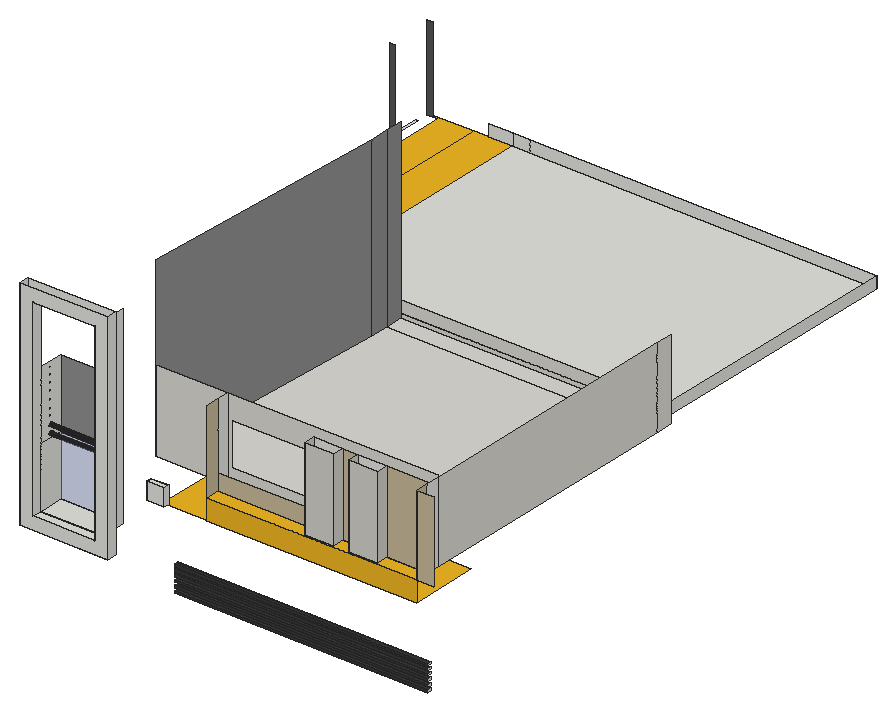
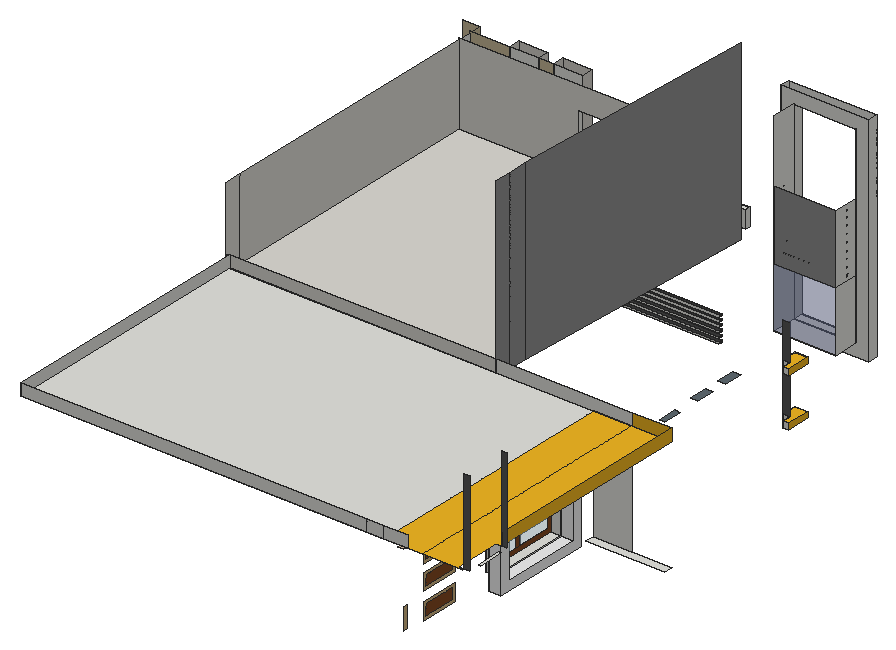
# SketchUp Ruby script. Lengths in inches.
U = 1.inch
M = Sketchup.active_model
def pt(a) = Geom::Point3d.new(a.map { |v| v * U })
def face(e, loops, mat)
  f = e.add_face(loops[0].map { |a| pt(a) })
  loops[1..].each { |l| e.add_face(l.map { |a| pt(a) }).erase! }
  f.material = f.back_material = mat if mat
  f
end
# faces: each face lists its corners as indices into pts; further lists are holes
def faces(e, pts, list, mat = nil) = list.each { |f| face(e, (f[0].is_a?(Array) ? f : [f]).map { |l| l.map { |i| pts[i] } }, mat) }
# xy, xz, yz: faces in a plane at the given z, y or x. An outline is a flat list of corners, or four numbers for a rectangle; further outlines are holes
def ring(l) = l.size == 4 ? [[l[0], l[1]], [l[2], l[1]], [l[2], l[3]], [l[0], l[3]]] : l.each_slice(2).to_a
def flat(e, list, mat, &to3) = list.each { |f| face(e, (f[0].is_a?(Array) ? f : [f]).map { |l| ring(l).map { |u, v| to3.(u, v) } }, mat) }
def xy(e, z, list, mat = nil) = flat(e, list, mat) { |x, y| [x, y, z] }
def xz(e, y, list, mat = nil) = flat(e, list, mat) { |x, z| [x, y, z] }
def yz(e, x, list, mat = nil) = flat(e, list, mat) { |y, z| [x, y, z] }
def lines(e, pts, list) = list.each { |a, b| e.add_line(pt(pts[a]), pt(pts[b])) }
# prism: a flat outline (further loops are holes) pulled along v
def prism(e, loops, v, mat = nil)
  f = face(e, loops, mat); d = Geom::Vector3d.new(v.map { |x| x * U })
  f.pushpull(f.normal.samedirection?(d) ? d.length : -d.length)
end
def box(e, o, s, mat = nil) = prism(e, [[o, [o[0] + s[0], o[1], o[2]], [o[0] + s[0], o[1] + s[1], o[2]], [o[0], o[1] + s[1], o[2]]]], [0, 0, s[2]], mat)
def at(x, y, z, deg = 0) = Geom::Transformation.translation(pt([x, y, z])) * Geom::Transformation.rotation(ORIGIN, Z_AXIS, deg.degrees)
def axes(o, x, y, z) = Geom::Transformation.new([*x, 0, *y, 0, *z, 0, *pt(o).to_a, 1])
def part(name) = M.definitions.add(name)
# library, detail: a bought-in or finely detailed component or shape, given as its bounding box
def library(name, o, s) = part(name).tap { |d| box(d.entities, o, s) }
def detail(e, o, s) = box(e.add_group.entities, o, s)
def put(e, d, t, mat = nil) = e.add_instance(d, t).tap { |i| i.material = mat if mat }
def group(e, t, mat = nil) = e.add_group.tap { |g| g.transformation = t; g.material = mat if mat }.entities
root = M.entities
M.materials.add("[0045_Goldenrod]").color = [239, 181, 35]
M.materials.add("[Carrera Marble]").color = [239, 239, 239]
M.materials.add("[Color M04]").color = [142, 142, 142]
M.materials.add("[Color M06]").color = [86, 86, 86]
M.materials.add("[Color M07]").color = [58, 58, 58]
M.materials.add("[Formica Laminate Light]").color = [213, 189, 164]
M.materials.add("[Formica Speckled Grey]").color = [94, 105, 111]
M.materials.add("[Quartz Light Brown]").color = [199, 184, 152]
M.materials.add("[Terrazzo Tile Light]").color = [219, 217, 210]
M.materials.add("[Tile Travertine 2 inch]").color = [211, 208, 201]
M.materials.add("[Translucent Glass Safety]").color = [204, 235, 244]
M.materials["[Translucent Glass Safety]"].alpha = 0.5
M.materials.add("[Translucent Glass Sky Reflection]").color = [126, 138, 183]
M.materials["[Translucent Glass Sky Reflection]"].alpha = 0.52
M.materials.add("[Wood Cherry Original]").color = [130, 73, 35]
M.materials.add("[Wood Floor Light]").color = [204, 176, 127]
box(root,[220.22,108.25,362.15],[19.63,5.9375,19.63])
xy(root,255.625,[[8.375,483.625,97.02,493.85]])
xy(root,256.33,[[226.34,139.81,513.45,143.95]])
xy(root,258.89,[[226.34,139.81,513.45,143.95]],"[Color M07]")
xy(root,261.64,[[226.34,139.81,513.45,143.95]])
xy(root,264.2,[[226.34,139.81,513.45,143.95]],"[Color M07]")
xy(root,265.95,[[82.9,518.89,97.02,632.14]],"[Carrera Marble]")
xy(root,267.45,[[226.34,139.81,513.45,143.95]])
xy(root,270.02,[[226.34,139.81,513.45,143.95]],"[Color M07]")
xy(root,273.08,[[226.34,139.81,513.45,143.95]])
xy(root,275.64,[[226.34,139.81,513.45,143.95]],"[Color M07]")
xy(root,276.41,[[97.02,529.35,108.15,621.68]])
xy(root,276.41,[[82.9,529.35,97.02,621.68]],"[Carrera Marble]")
xy(root,278.27,[[226.34,139.81,513.45,143.95]])
xy(root,280.83,[[226.34,139.81,513.45,143.95]],"[Color M07]")
xy(root,283.14,[[226.34,139.81,513.45,143.95]])
xy(root,283.375,[[73.3,112.625,172.24,123.625]])
xy(root,285.7,[[226.34,139.81,513.45,143.95]],"[Color M07]")
xy(root,295.16,[[38.625,253.03,38.625,280.03,45.3125,280.03,45.3125,270.46,53.375,270.46,53.375,253.03]],"[0045_Goldenrod]")
xy(root,297.39,[[87.31,112.625,158.23,123.625],[87.31,123.625,158.23,152]])
xy(root,301.97,[[38.625,253.03,53.375,253.03,53.375,270.46,45.3125,270.46,45.3125,280.03,38.625,280.03]],"[0045_Goldenrod]")
xy(root,350.16,[[38.625,253.03,38.625,280.03,45.3125,280.03,45.3125,270.46,53.375,270.46,53.375,253.03]],"[0045_Goldenrod]")
xy(root,354.51,[[226.34,123.625,513.45,200.74]],"[0045_Goldenrod]")
xy(root,356.97,[[38.625,253.03,53.375,253.03,53.375,270.46,45.3125,270.46,45.3125,280.03,38.625,280.03]],"[0045_Goldenrod]")
xy(root,358.98,[[82.9,529.35,97.02,621.68],[97.02,529.35,108.15,621.68]])
xy(root,360.75,[[97.02,660.4,103.59,752.02]],"[Formica Laminate Light]")
xy(root,367.23,[[53.375,329.31,62.1875,350.56],[53.375,368.62,61.9375,389.87],[53.375,415.62,59.375,436.87]],"[Formica Speckled Grey]")
xy(root,369.45,[[82.9,518.89,97.02,632.14]],"[Carrera Marble]")
xy(root,378,[[435.42,123.625,467.86,125.375],[385.17,125.375,418.48,138.52],[435.42,125.375,467.86,138.52],[276.16,138.52,513.45,153.42]])
xy(root,378,[[276.16,123.625,435.42,123.625,435.42,138.52,418.48,138.52,418.48,125.375,385.17,125.375,385.17,138.52,276.16,138.52],[467.86,123.625,513.45,138.52]],"[0045_Goldenrod]")
xy(root,378,[[194.63,153.42,513.45,153.42,513.45,463.7,208.03,463.7,208.03,442.17],[208.03,463.7,513.45,483.625]],"[Terrazzo Tile Light]")
xy(root,383.375,[[97.02,483.625,509.21,779.875]])
xy(root,383.375,[[8.375,483.625,8.375,724.47,14.37,724.47,14.37,777.2,8.375,777.2,8.375,779.875,53.375,779.875,53.375,483.625],[53.375,483.625,97.02,779.875]],"[0045_Goldenrod]")
xy(root,383.48,[[0,735.45,2.5625,763.82]])
xz(root,112.625,[[[73.3,283.375,172.24,529.3125],[87.31,297.39,158.23,515.31]]])
xz(root,123.625,[[[73.3,283.375,172.24,529.3125],[87.31,297.39,158.23,515.31]]])
xz(root,123.625,[[276.16,354.51,513.45,378]],"[0045_Goldenrod]")
xz(root,123.625,[[513.45,378,533.375,468.5]],"[Quartz Light Brown]")
xz(root,125.375,[[385.17,378,418.48,471],[435.42,378,467.86,471]],"[Tile Travertine 2 inch]")
xz(root,138.52,[[385.17,378,418.48,471],[435.42,378,467.86,471]])
xz(root,138.52,[[276.16,378,385.17,396.69],[418.48,378,435.42,471],[467.86,378,513.45,471]],"[Quartz Light Brown]")
xz(root,139.81,[[226.34,256.33,513.45,258.89],[226.34,261.64,513.45,264.2],[226.34,267.45,513.45,270.02],[226.34,273.08,513.45,275.64],[226.34,278.27,513.45,280.83],
  [226.34,283.14,513.45,285.7]],"[Color M07]")
xz(root,143.95,[[226.34,256.33,513.45,258.89],[226.34,261.64,513.45,264.2],[226.34,267.45,513.45,270.02],[226.34,273.08,513.45,275.64],[226.34,278.27,513.45,280.83],
  [226.34,283.14,513.45,285.7]])
xz(root,152,[[87.31,365.69,158.23,444.16]],"[Color M04]")
xz(root,152,[[87.31,297.39,158.23,365.69]],"[Translucent Glass Sky Reflection]")
xz(root,153.42,[[194.63,378,276.16,471],[[276.16,378,513.45,471],[280.22,396.69,379.09,445.19]]],"[Terrazzo Tile Light]")
xz(root,253.03,[[38.625,295.16,53.375,301.97],[38.625,350.16,53.375,356.97]],"[0045_Goldenrod]")
xz(root,270.46,[[45.3125,295.16,53.375,301.97],[45.3125,350.16,53.375,356.97]])
xz(root,270.46,[[45.3125,301.97,53.375,350.16],[45.3125,356.97,53.375,397.66]],"[Color M06]")
xz(root,280.03,[[38.625,295.16,45.3125,301.97],[38.625,350.16,45.3125,356.97]])
xz(root,483.625,[[53.375,255.625,97.02,383.375],[509.21,378,513.45,396.875],[53.375,383.375,208.03,396.875]])
xz(root,483.625,[[8.375,383.375,53.375,396.875]],"[0045_Goldenrod]")
xz(root,483.625,[[208.03,378,509.21,383.375],[208.03,383.375,509.21,396.875]],"[Terrazzo Tile Light]")
xz(root,518.89,[[82.9,265.95,97.02,369.45]],"[Carrera Marble]")
xz(root,529.35,[[97.02,276.41,108.15,358.98]])
xz(root,529.35,[[82.9,276.41,97.02,358.98]],"[Carrera Marble]")
xz(root,621.68,[[97.02,276.41,108.15,358.98]])
xz(root,621.68,[[82.9,276.41,97.02,358.98]],"[Carrera Marble]")
xz(root,632.14,[[82.9,265.95,97.02,369.45]],"[Carrera Marble]")
xz(root,724.47,[[2.5625,383.375,8.375,479.1875]],"[Color M06]")
xz(root,777.2,[[2.5625,383.375,8.375,479.1875]],"[Color M06]")
xz(root,779.875,[[70.21,383.375,97.02,396.875],[97.02,383.375,116.75,396.875],[116.75,383.375,509.21,396.875]])
yz(root,8.375,[[483.625,383.375,724.47,396.875]],"[0045_Goldenrod]")
yz(root,38.625,[[253.03,295.16,280.03,301.97],[253.03,350.16,280.03,356.97]],"[0045_Goldenrod]")
yz(root,45.3125,[[270.46,295.16,280.03,301.97],[270.46,350.16,280.03,356.97]])
yz(root,53.375,[[253.03,295.16,270.46,301.97],[253.03,350.16,270.46,356.97]])
yz(root,73.3,[[112.625,283.375,123.625,529.3125]])
yz(root,82.9,[[[518.89,265.95,632.14,369.45],[529.35,276.41,621.68,358.98]]],"[Carrera Marble]")
yz(root,87.31,[[112.625,297.39,123.625,515.31],[123.625,297.39,152,365.69],[[123.625,365.69,152,444.16],[136.99,436.55,136.55,436.61,136.14,436.78,135.79,437.05,135.52,437.4,135.36,437.81,135.3,438.24,135.36,438.68,135.52,439.09,135.79,439.44,136.14,439.7,136.55,439.87,136.99,439.93,137.42,439.87,137.83,439.7,138.18,439.44,138.45,439.09,138.62,438.68,138.67,438.24,138.62,437.81,138.45,437.4,138.18,437.05,137.83,436.78,137.42,436.61],[136.99,369.93,136.55,369.99,136.14,370.16,135.79,370.42,135.52,370.77,135.36,371.18,135.3,371.62,135.36,372.05,135.52,372.46,135.79,372.81,136.14,373.08,136.55,373.25,136.99,373.3,137.42,373.25,137.83,373.08,138.18,372.81,138.45,372.46,138.62,372.05,138.67,371.62,138.62,371.18,138.45,370.77,138.18,370.42,137.83,370.16,137.42,369.99],[136.99,429.05,136.55,429.11,136.14,429.28,135.79,429.55,135.52,429.9,135.36,430.31,135.3,430.74,135.36,431.18,135.52,431.59,135.79,431.94,136.14,432.2,136.55,432.37,136.99,432.43,137.42,432.37,137.83,432.2,138.18,431.94,138.45,431.59,138.62,431.18,138.67,430.74,138.62,430.31,138.45,429.9,138.18,429.55,137.83,429.28,137.42,429.11],[136.99,378.62,136.55,378.67,136.14,378.84,135.79,379.11,135.52,379.46,135.36,379.87,135.3,380.3,135.36,380.74,135.52,381.15,135.79,381.5,136.14,381.77,136.55,381.93,136.99,381.99,137.42,381.93,137.83,381.77,138.18,381.5,138.45,381.15,138.62,380.74,138.67,380.3,138.62,379.87,138.45,379.46,138.18,379.11,137.83,378.84,137.42,378.67],[136.99,420.74,136.55,420.8,136.14,420.97,135.79,421.24,135.52,421.59,135.36,421.99,135.3,422.43,135.36,422.87,135.52,423.27,135.79,423.62,136.14,423.89,136.55,424.06,136.99,424.12,137.42,424.06,137.83,423.89,138.18,423.62,138.45,423.27,138.62,422.87,138.67,422.43,138.62,421.99,138.45,421.59,138.18,421.24,137.83,420.97,137.42,420.8],[136.99,387.18,136.55,387.24,136.14,387.41,135.79,387.67,135.52,388.02,135.36,388.43,135.3,388.87,135.36,389.3,135.52,389.71,135.79,390.06,136.14,390.33,136.55,390.5,136.99,390.55,137.42,390.5,137.83,390.33,138.18,390.06,138.45,389.71,138.62,389.3,138.67,388.87,138.62,388.43,138.45,388.02,138.18,387.67,137.83,387.41,137.42,387.24],[136.99,412.55,136.55,412.61,136.14,412.78,135.79,413.05,135.52,413.4,135.36,413.81,135.3,414.24,135.36,414.68,135.52,415.09,135.79,415.44,136.14,415.7,136.55,415.87,136.99,415.93,137.42,415.87,137.83,415.7,138.18,415.44,138.45,415.09,138.62,414.68,138.67,414.24,138.62,413.81,138.45,413.4,138.18,413.05,137.83,412.78,137.42,412.61],[136.99,394.8,136.55,394.86,136.14,395.03,135.79,395.3,135.52,395.65,135.36,396.06,135.3,396.49,135.36,396.93,135.52,397.34,135.79,397.69,136.14,397.95,136.55,398.12,136.99,398.18,137.42,398.12,137.83,397.95,138.18,397.69,138.45,397.34,138.62,396.93,138.67,396.49,138.62,396.06,138.45,395.65,138.18,395.3,137.83,395.03,137.42,394.86],[136.99,403.55,136.55,403.61,136.14,403.78,135.79,404.05,135.52,404.4,135.36,404.81,135.3,405.24,135.36,405.68,135.52,406.09,135.79,406.44,136.14,406.7,136.55,406.87,136.99,406.93,137.42,406.87,137.83,406.7,138.18,406.44,138.45,406.09,138.62,405.68,138.67,405.24,138.62,404.81,138.45,404.4,138.18,404.05,137.83,403.78,137.42,403.61]],[136.99,369.93,136.55,369.99,136.14,370.16,135.79,370.42,135.52,370.77,135.36,371.18,135.3,371.62,135.36,372.05,135.52,372.46,135.79,372.81,136.14,373.08,136.55,373.25,136.99,373.3,137.42,373.25,137.83,373.08,138.18,372.81,138.45,372.46,138.62,372.05,138.67,371.62,138.62,371.18,138.45,370.77,138.18,370.42,137.83,370.16,137.42,369.99],[136.99,378.62,136.55,378.67,136.14,378.84,135.79,379.11,135.52,379.46,135.36,379.87,135.3,380.3,135.36,380.74,135.52,381.15,135.79,381.5,136.14,381.77,136.55,381.93,136.99,381.99,137.42,381.93,137.83,381.77,138.18,381.5,138.45,381.15,138.62,380.74,138.67,380.3,138.62,379.87,138.45,379.46,138.18,379.11,137.83,378.84,137.42,378.67]])
yz(root,97.02,[[[518.89,265.95,632.14,369.45],[529.35,276.41,621.68,358.98]]])
yz(root,103.59,[[675.22,273.32,712.4,285.1875],[675.22,303.38,712.4,315.25],[675.22,331.38,712.4,343.25]],"[Wood Cherry Original]")
yz(root,103.59,[[[671.74,269.85,715.87,288.66],[675.22,273.32,712.4,285.1875]],[739.76,272.3,743.82,296.74],[[671.74,299.91,715.87,318.72],[675.22,303.38,712.4,315.25]],[[671.74,327.91,715.87,346.72],[675.22,331.38,712.4,343.25]]],"[Wood Floor Light]")
yz(root,108.15,[[534.55,281.61,573.77,353.78],[580.2,281.61,616.48,353.78]],"[Translucent Glass Safety]")
yz(root,108.15,[[[529.35,276.41,621.68,358.98],[534.55,281.61,616.48,353.78]],[573.77,281.61,580.2,353.78]],"[Wood Cherry Original]")
yz(root,158.23,[[112.625,297.39,123.625,515.31],[[123.625,297.39,152,515.31],[136.99,436.55,137.42,436.61,137.83,436.78,138.18,437.05,138.45,437.4,138.62,437.81,138.67,438.24,138.62,438.68,138.45,439.09,138.18,439.44,137.83,439.7,137.42,439.87,136.99,439.93,136.55,439.87,136.14,439.7,135.79,439.44,135.52,439.09,135.36,438.68,135.3,438.24,135.36,437.81,135.52,437.4,135.79,437.05,136.14,436.78,136.55,436.61],[136.99,429.05,137.42,429.11,137.83,429.28,138.18,429.55,138.45,429.9,138.62,430.31,138.67,430.74,138.62,431.18,138.45,431.59,138.18,431.94,137.83,432.2,137.42,432.37,136.99,432.43,136.55,432.37,136.14,432.2,135.79,431.94,135.52,431.59,135.36,431.18,135.3,430.74,135.36,430.31,135.52,429.9,135.79,429.55,136.14,429.28,136.55,429.11],[136.99,420.74,137.42,420.8,137.83,420.97,138.18,421.24,138.45,421.59,138.62,421.99,138.67,422.43,138.62,422.87,138.45,423.27,138.18,423.62,137.83,423.89,137.42,424.06,136.99,424.12,136.55,424.06,136.14,423.89,135.79,423.62,135.52,423.27,135.36,422.87,135.3,422.43,135.36,421.99,135.52,421.59,135.79,421.24,136.14,420.97,136.55,420.8],[136.99,412.55,137.42,412.61,137.83,412.78,138.18,413.05,138.45,413.4,138.62,413.81,138.67,414.24,138.62,414.68,138.45,415.09,138.18,415.44,137.83,415.7,137.42,415.87,136.99,415.93,136.55,415.87,136.14,415.7,135.79,415.44,135.52,415.09,135.36,414.68,135.3,414.24,135.36,413.81,135.52,413.4,135.79,413.05,136.14,412.78,136.55,412.61],[136.99,403.55,137.42,403.61,137.83,403.78,138.18,404.05,138.45,404.4,138.62,404.81,138.67,405.24,138.62,405.68,138.45,406.09,138.18,406.44,137.83,406.7,137.42,406.87,136.99,406.93,136.55,406.87,136.14,406.7,135.79,406.44,135.52,406.09,135.36,405.68,135.3,405.24,135.36,404.81,135.52,404.4,135.79,404.05,136.14,403.78,136.55,403.61],[136.99,394.8,137.42,394.86,137.83,395.03,138.18,395.3,138.45,395.65,138.62,396.06,138.67,396.49,138.62,396.93,138.45,397.34,138.18,397.69,137.83,397.95,137.42,398.12,136.99,398.18,136.55,398.12,136.14,397.95,135.79,397.69,135.52,397.34,135.36,396.93,135.3,396.49,135.36,396.06,135.52,395.65,135.79,395.3,136.14,395.03,136.55,394.86],[136.99,387.18,137.42,387.24,137.83,387.41,138.18,387.67,138.45,388.02,138.62,388.43,138.67,388.87,138.62,389.3,138.45,389.71,138.18,390.06,137.83,390.33,137.42,390.5,136.99,390.55,136.55,390.5,136.14,390.33,135.79,390.06,135.52,389.71,135.36,389.3,135.3,388.87,135.36,388.43,135.52,388.02,135.79,387.67,136.14,387.41,136.55,387.24],[136.99,378.62,137.42,378.67,137.83,378.84,138.18,379.11,138.45,379.46,138.62,379.87,138.67,380.3,138.62,380.74,138.45,381.15,138.18,381.5,137.83,381.77,137.42,381.93,136.99,381.99,136.55,381.93,136.14,381.77,135.79,381.5,135.52,381.15,135.36,380.74,135.3,380.3,135.36,379.87,135.52,379.46,135.79,379.11,136.14,378.84,136.55,378.67],[136.99,369.93,137.42,369.99,137.83,370.16,138.18,370.42,138.45,370.77,138.62,371.18,138.67,371.62,138.62,372.05,138.45,372.46,138.18,372.81,137.83,373.08,137.42,373.25,136.99,373.3,136.55,373.25,136.14,373.08,135.79,372.81,135.52,372.46,135.36,372.05,135.3,371.62,135.36,371.18,135.52,370.77,135.79,370.42,136.14,370.16,136.55,369.99]]])
yz(root,172.24,[[112.625,283.375,123.625,529.3125]])
yz(root,208.03,[[442.17,378,463.7,577.3125],[463.7,378,483.625,577.3125]],"[Color M04]")
yz(root,276.16,[[138.52,378,153.42,471]])
yz(root,276.16,[[123.625,378,138.52,471]],"[Quartz Light Brown]")
yz(root,385.17,[[125.375,378,138.52,471]],"[Tile Travertine 2 inch]")
yz(root,418.48,[[125.375,378,138.52,471]],"[Tile Travertine 2 inch]")
yz(root,435.42,[[125.375,378,138.52,471]],"[Tile Travertine 2 inch]")
yz(root,467.86,[[125.375,378,138.52,471]],"[Tile Travertine 2 inch]")
yz(root,509.21,[[483.625,383.375,779.875,396.875]])
yz(root,513.45,[[139.81,256.33,143.95,258.89],[139.81,261.64,143.95,264.2],[139.81,267.45,143.95,270.02],[139.81,273.08,143.95,275.64],[139.81,278.27,143.95,280.83],
  [139.81,283.14,143.95,285.7],[138.52,378,153.42,468.5]])
yz(root,513.45,[[123.625,378,138.52,468.5]],"[Quartz Light Brown]")
yz(root,513.45,[[153.42,378,463.7,468.5],[463.7,378,483.625,468.5]],"[Terrazzo Tile Light]")
p = [[87.31,136.55,369.99],[87.31,136.99,369.93],[158.23,136.99,369.93],[158.23,136.55,369.99],[87.31,137.42,369.99],[158.23,137.42,369.99],
  [87.31,136.14,370.16],[158.23,136.14,370.16],[87.31,137.83,370.16],[158.23,137.83,370.16],[87.31,135.79,370.42],[158.23,135.79,370.42],
  [87.31,138.18,370.42],[158.23,138.18,370.42],[87.31,135.52,370.77],[158.23,135.52,370.77],[87.31,138.45,370.77],[158.23,138.45,370.77],
  [87.31,135.36,371.18],[158.23,135.36,371.18],[87.31,138.62,371.18],[158.23,138.62,371.18],[87.31,135.3,371.62],[158.23,135.3,371.62],
  [87.31,138.67,371.62],[158.23,138.67,371.62],[87.31,135.36,372.05],[158.23,135.36,372.05],[87.31,138.62,372.05],[158.23,138.62,372.05],
  [87.31,135.52,372.46],[158.23,135.52,372.46],[87.31,138.45,372.46],[158.23,138.45,372.46],[87.31,135.79,372.81],[158.23,135.79,372.81],
  [87.31,138.18,372.81],[158.23,138.18,372.81],[87.31,136.14,373.08],[158.23,136.14,373.08],[87.31,137.83,373.08],[158.23,137.83,373.08],
  [87.31,136.55,373.25],[158.23,136.55,373.25],[87.31,137.42,373.25],[158.23,137.42,373.25],[87.31,136.99,373.3],[158.23,136.99,373.3],
  [194.63,153.42,378],[208.03,442.17,378],[208.03,442.17,577.3125],[194.63,153.42,577.3125],[194.63,153.42,481.9375],[194.63,153.42,471],
  [87.31,136.55,378.67],[87.31,136.99,378.62],[158.23,136.99,378.62],[158.23,136.55,378.67],[87.31,137.42,378.67],[158.23,137.42,378.67],
  [87.31,136.14,378.84],[158.23,136.14,378.84],[87.31,137.83,378.84],[158.23,137.83,378.84],[87.31,135.79,379.11],[158.23,135.79,379.11],
  [87.31,138.18,379.11],[158.23,138.18,379.11],[87.31,135.52,379.46],[158.23,135.52,379.46],[87.31,138.45,379.46],[158.23,138.45,379.46],
  [87.31,135.36,379.87],[158.23,135.36,379.87],[87.31,138.62,379.87],[158.23,138.62,379.87],[87.31,135.3,380.3],[158.23,135.3,380.3],
  [87.31,138.67,380.3],[158.23,138.67,380.3],[87.31,135.36,380.74],[158.23,135.36,380.74],[87.31,138.62,380.74],[158.23,138.62,380.74],
  [87.31,135.52,381.15],[158.23,135.52,381.15],[87.31,138.45,381.15],[158.23,138.45,381.15],[87.31,135.79,381.5],[158.23,135.79,381.5],
  [87.31,138.18,381.5],[158.23,138.18,381.5],[87.31,136.14,381.77],[158.23,136.14,381.77],[87.31,137.83,381.77],[158.23,137.83,381.77],
  [87.31,136.55,381.93],[158.23,136.55,381.93],[87.31,137.42,381.93],[158.23,137.42,381.93],[87.31,136.99,381.99],[158.23,136.99,381.99]]
faces(root,p,[[0,1,2,3],[1,4,5,2],[6,0,3,7],[4,8,9,5],[10,6,7,11],[8,12,13,9],[14,10,11,15],[12,16,17,13],
  [18,14,15,19],[16,20,21,17],[22,18,19,23],[20,24,25,21],[26,22,23,27],[24,28,29,25],[30,26,27,31],[28,32,33,29],
  [34,30,31,35],[32,36,37,33],[38,34,35,39],[36,40,41,37],[42,38,39,43],[40,44,45,41],[46,42,43,47],[44,46,47,45],
  [54,55,56,57],[55,58,59,56],[60,54,57,61],[58,62,63,59],[64,60,61,65],[62,66,67,63],[68,64,65,69],[66,70,71,67],
  [72,68,69,73],[70,74,75,71],[76,72,73,77],[74,78,79,75],[80,76,77,81],[78,82,83,79],[84,80,81,85],[82,86,87,83],
  [88,84,85,89],[86,90,91,87],[92,88,89,93],[90,94,95,91],[96,92,93,97],[94,98,99,95],[100,96,97,101],[98,100,101,99]],"[Color M07]")
faces(root,p,[[48,49,50,51,52,53]],"[Color M04]")
